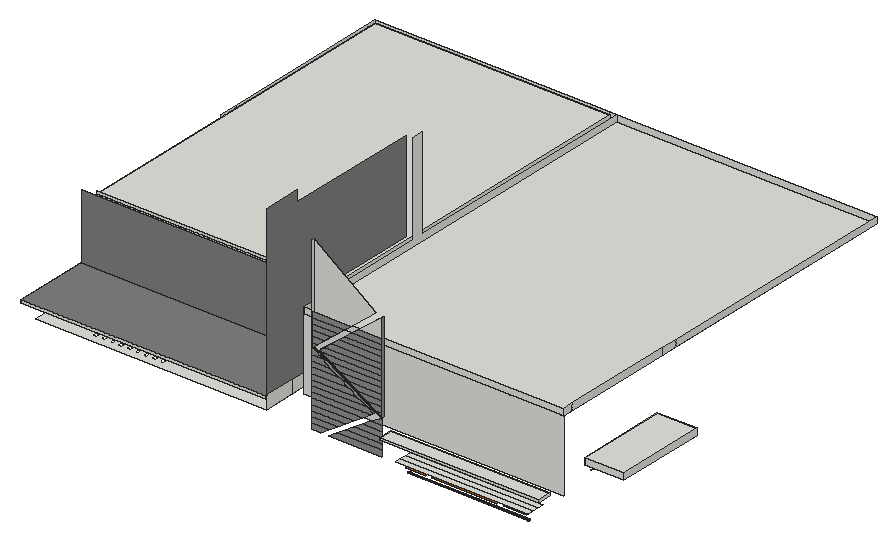
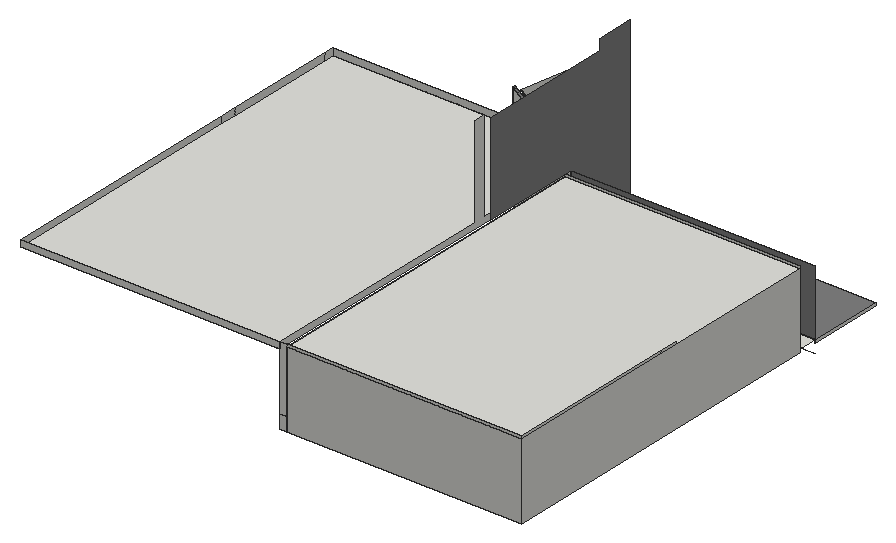
# SketchUp Ruby script. Lengths in inches.
U = 1.inch
M = Sketchup.active_model
def pt(a) = Geom::Point3d.new(a.map { |v| v * U })
def face(e, loops, mat)
  f = e.add_face(loops[0].map { |a| pt(a) })
  loops[1..].each { |l| e.add_face(l.map { |a| pt(a) }).erase! }
  f.material = f.back_material = mat if mat
  f
end
# faces: each face lists its corners as indices into pts; further lists are holes
def faces(e, pts, list, mat = nil) = list.each { |f| face(e, (f[0].is_a?(Array) ? f : [f]).map { |l| l.map { |i| pts[i] } }, mat) }
# xy, xz, yz: faces in a plane at the given z, y or x. An outline is a flat list of corners, or four numbers for a rectangle; further outlines are holes
def ring(l) = l.size == 4 ? [[l[0], l[1]], [l[2], l[1]], [l[2], l[3]], [l[0], l[3]]] : l.each_slice(2).to_a
def flat(e, list, mat, &to3) = list.each { |f| face(e, (f[0].is_a?(Array) ? f : [f]).map { |l| ring(l).map { |u, v| to3.(u, v) } }, mat) }
def xy(e, z, list, mat = nil) = flat(e, list, mat) { |x, y| [x, y, z] }
def xz(e, y, list, mat = nil) = flat(e, list, mat) { |x, z| [x, y, z] }
def yz(e, x, list, mat = nil) = flat(e, list, mat) { |y, z| [x, y, z] }
def lines(e, pts, list) = list.each { |a, b| e.add_line(pt(pts[a]), pt(pts[b])) }
# prism: a flat outline (further loops are holes) pulled along v
def prism(e, loops, v, mat = nil)
  f = face(e, loops, mat); d = Geom::Vector3d.new(v.map { |x| x * U })
  f.pushpull(f.normal.samedirection?(d) ? d.length : -d.length)
end
def box(e, o, s, mat = nil) = prism(e, [[o, [o[0] + s[0], o[1], o[2]], [o[0] + s[0], o[1] + s[1], o[2]], [o[0], o[1] + s[1], o[2]]]], [0, 0, s[2]], mat)
def at(x, y, z, deg = 0) = Geom::Transformation.translation(pt([x, y, z])) * Geom::Transformation.rotation(ORIGIN, Z_AXIS, deg.degrees)
def axes(o, x, y, z) = Geom::Transformation.new([*x, 0, *y, 0, *z, 0, *pt(o).to_a, 1])
def part(name) = M.definitions.add(name)
# library, detail: a bought-in or finely detailed component or shape, given as its bounding box
def library(name, o, s) = part(name).tap { |d| box(d.entities, o, s) }
def detail(e, o, s) = box(e.add_group.entities, o, s)
def put(e, d, t, mat = nil) = e.add_instance(d, t).tap { |i| i.material = mat if mat }
def group(e, t, mat = nil) = e.add_group.tap { |g| g.transformation = t; g.material = mat if mat }.entities
root = M.entities
M.materials.add("[0132_LightGray]").color = [169, 169, 169]
M.materials.add("[0133_Gray]").color = [128, 128, 128]
M.materials.add("[Color M04]").color = [142, 142, 142]
M.materials.add("[Wood Bamboo]").color = [195, 96, 5]
xy(root,318.58,[[351.24,38.65,369.24,44.67],[375.24,38.65,435.1,44.67],[441.1,38.65,462.7,44.67]],"[Wood Bamboo]")
xy(root,323.97,[[345.84,33.25,468.09,38.65],[345.84,38.65,468.09,44.67],[345.84,44.67,468.09,50.6875]])
xy(root,337.75,[[332.44,31.5625,478.87,33.25],[332.44,33.25,333.13,44.6875],[333.13,33.25,478.31,44.6875],[478.31,33.25,478.87,44.6875]])
xy(root,338,[[[28.03,15.6875,241.25,84.25],[55.53,37.52,56.5625,37.65,57.53,38.05,58.36,38.6875,58.99,39.52,59.39,40.48,59.53,41.52,59.39,42.55,58.99,43.52,58.36,44.34,57.53,44.98,56.5625,45.38,55.53,45.52,54.49,45.38,53.53,44.98,52.7,44.34,52.0625,43.52,51.66,42.55,51.53,41.52,51.66,40.48,52.0625,39.52,52.7,38.6875,53.53,38.05,54.49,37.65],[198.34,37.52,199.375,37.65,200.34,38.05,201.17,38.6875,201.8,39.52,202.2,40.48,202.34,41.52,202.2,42.55,201.8,43.52,201.17,44.34,200.34,44.98,199.375,45.38,198.34,45.52,197.31,45.38,196.34,44.98,195.51,44.34,194.875,43.52,194.48,42.55,194.34,41.52,194.48,40.48,194.875,39.52,195.51,38.6875,196.34,38.05,197.31,37.65],[74.77,23.01,78.7,26.95],[82.52,23.01,86.45,26.95],[90.27,23.01,94.2,26.95],[98.02,23.01,101.95,26.95],[105.77,23.01,109.7,26.95],[113.52,23.01,117.45,26.95],[121.27,23.01,125.2,26.95],[129.02,23.01,132.95,26.95],[136.77,23.01,140.7,26.95]],[55.53,37.52,54.49,37.65,53.53,38.05,52.7,38.6875,52.0625,39.52,51.66,40.48,51.53,41.52,51.66,42.55,52.0625,43.52,52.7,44.34,53.53,44.98,54.49,45.38,55.53,45.52,56.5625,45.38,57.53,44.98,58.36,44.34,58.99,43.52,59.39,42.55,59.53,41.52,59.39,40.48,58.99,39.52,58.36,38.6875,57.53,38.05,56.5625,37.65],[198.34,37.52,197.31,37.65,196.34,38.05,195.51,38.6875,194.875,39.52,194.48,40.48,194.34,41.52,194.48,42.55,194.875,43.52,195.51,44.34,196.34,44.98,197.31,45.38,198.34,45.52,199.375,45.38,200.34,44.98,201.17,44.34,201.8,43.52,202.2,42.55,202.34,41.52,202.2,40.48,201.8,39.52,201.17,38.6875,200.34,38.05,199.375,37.65]])
xy(root,339.8125,[[332.44,31.5625,478.87,44.6875]])
xy(root,347,[[14.875,14.6875,14.875,84.25,15.875,84.25,15.875,15.6875,241.25,15.6875,241.25,14.6875]])
xy(root,350,[[14.875,14.6875,241.25,84.25]],"[0133_Gray]")
xy(root,354,[[495.875,70.375,496.875,140.375]])
xy(root,361,[[495.875,63.375,496.875,147.375],[[496.875,63.375,531.875,147.375],[514.17,93.74,515.73,93.95,517.17,94.55,518.42,95.5,519.37,96.74,519.97,98.1875,520.17,99.74,519.97,101.3,519.37,102.74,518.42,103.98,517.17,104.9375,515.73,105.54,514.17,105.74,512.62,105.54,511.17,104.9375,509.93,103.98,508.98,102.74,508.375,101.3,508.17,99.74,508.375,98.1875,508.98,96.74,509.93,95.5,511.17,94.55,512.62,93.95]],[514.17,93.74,512.62,93.95,511.17,94.55,509.93,95.5,508.98,96.74,508.375,98.1875,508.17,99.74,508.375,101.3,508.98,102.74,509.93,103.98,511.17,104.9375,512.62,105.54,514.17,105.74,515.73,105.54,517.17,104.9375,518.42,103.98,519.37,102.74,519.97,101.3,520.17,99.74,519.97,98.1875,519.37,96.74,518.42,95.5,517.17,94.55,515.73,93.95]])
xy(root,367,[[495.875,63.375,531.875,147.375]])
xy(root,404,[[247.25,50.6875,486.875,411]])
xy(root,407.75,[[24.875,90.25,241.25,411]])
xz(root,14.6875,[[14.875,347,241.25,350]])
xz(root,31.5625,[[332.44,337.75,478.87,339.8125]])
xz(root,42.75,[[261.37,317.04,269.28,317.04,276.97,322.17,261.37,322.17],[276.6875,317.04,325.49,317.04,325.49,322.17,284.48,322.17],[261.37,322.17,276.97,322.17,284.66,327.29,261.37,327.29],[284.48,322.17,325.49,322.17,325.49,327.29,292.26,327.29],[261.37,327.29,284.66,327.29,292.35,332.42,261.37,332.42],
  [292.26,327.29,325.49,327.29,325.49,332.42,300.05,332.42],[261.37,332.42,292.35,332.42,300.04,337.54,261.37,337.54],[300.05,332.42,325.49,332.42,325.49,337.54,307.84,337.54],[261.37,337.54,300.04,337.54,307.73,342.67,261.37,342.67],[307.84,337.54,325.49,337.54,325.49,342.67,315.63,342.67],
  [261.37,342.67,307.73,342.67,315.42,347.79,261.37,347.79],[315.63,342.67,325.49,342.67,325.49,347.79,323.42,347.79],[261.37,347.79,315.42,347.79,317.38,349.1,311.37,352.92,261.37,352.92],[323.42,347.79,325.49,347.79,325.49,349.15],[325.49,349.15,325.49,352.92,319.41,352.92],
  [261.37,352.92,311.37,352.92,303.28,358.04,261.37,358.04],[319.41,352.92,325.49,352.92,325.49,358.04,311.14,358.04],[261.37,358.04,303.28,358.04,295.19,363.17,261.37,363.17],[311.14,358.04,325.49,358.04,325.49,363.17,302.875,363.17],[261.37,363.17,295.19,363.17,287.1,368.29,261.37,368.29],
  [302.875,363.17,325.49,363.17,325.49,368.29,294.61,368.29],[261.37,368.29,287.1,368.29,279.02,373.42,261.37,373.42],[294.61,368.29,325.49,368.29,325.49,373.42,286.34,373.42],[261.37,373.42,279.02,373.42,270.93,378.54,261.37,378.54],[286.34,373.42,325.49,373.42,325.49,378.54,278.07,378.54],
  [261.37,378.54,270.93,378.54,262.84,383.67,261.37,383.67],[278.07,378.54,325.49,378.54,325.49,383.67,269.8,383.67],[261.37,383.67,262.84,383.67,261.37,384.6],[269.8,383.67,325.49,383.67,325.49,388.79,273.37,388.79,268.3,384.6],[261.37,384.6,266.38,388.79,261.37,388.79],
  [261.37,388.79,266.38,388.79,272.51,393.92,261.37,393.92],[273.37,388.79,325.49,388.79,325.49,393.92,279.58,393.92],[261.37,393.92,272.51,393.92,278.64,399.04,261.37,399.04],[279.58,393.92,325.49,393.92,325.49,399.04,285.78,399.04],[261.37,399.04,278.64,399.04,284.76,404.17,261.37,404.17],
  [285.78,399.04,325.49,399.04,325.49,404.17,291.99,404.17],[261.37,404.17,284.76,404.17,290.89,409.29,261.37,409.29],[291.99,404.17,325.49,404.17,325.49,409.29,298.19,409.29],[261.37,409.29,290.89,409.29,297.02,414.42,261.37,414.42],[298.19,409.29,325.49,409.29,325.49,414.42,304.39,414.42]],"[Color M04]")
xz(root,44.6875,[[332.44,337.75,478.87,339.8125],[325.49,349.15,268.3,384.6,325.49,431.84],[261.37,384.6,261.37,473.32,318.21,432.15]])
xz(root,50.6875,[[247.25,338,486.875,404],[247.25,404,486.875,410]])
xz(root,63.375,[[495.875,361,531.875,367]])
xz(root,84.25,[[14.875,347,15.875,350]])
xz(root,84.25,[[15.875,350,241.25,410]],"[0133_Gray]")
xz(root,90.25,[[24.875,338,241.25,407.75],[24.875,407.75,241.25,410]])
xz(root,147.375,[[495.875,361,531.875,367]])
xz(root,411,[[24.875,338,241.25,407.75],[241.25,338,247.25,350],[241.25,350,247.25,410],[247.25,404,486.875,410],[24.875,407.75,241.25,410]])
yz(root,14.875,[[14.6875,347,84.25,350]])
yz(root,24.875,[[90.25,338,411,407.75],[233.22,407.75,250.625,410],[250.625,407.75,411,410]])
yz(root,241.25,[[15.6875,338,44.6875,350],[44.6875,338,84.25,350],[90.25,338,411,407.75],[14.6875,347,15.6875,350]])
yz(root,241.25,[[15.6875,350,15.6875,503.875,50.6875,503.875,50.6875,494,176.25,494,176.25,410,84.25,410,84.25,350]],"[0133_Gray]")
yz(root,247.25,[[50.6875,404,411,404,411,410,187,410,187,494,176.25,494,176.25,410,50.6875,410]])
yz(root,261.37,[[42.75,384.6,44.6875,473.32]])
yz(root,325.49,[[42.75,349.15,44.6875,431.84]],"[Color M04]")
yz(root,332.44,[[31.5625,337.75,44.6875,339.8125]])
yz(root,478.87,[[31.5625,337.75,44.6875,339.8125]])
yz(root,486.875,[[50.6875,404,60.17,410],[60.17,404,163.89,410],[163.89,404,180.07,410],[180.07,404,411,410]])
yz(root,495.875,[[63.375,361,147.375,367]])
yz(root,531.875,[[63.375,361,147.375,367]])
p = [[351.24,41.41,313.07],[351.24,41.53,313.02],[462.7,41.53,313.02],[462.7,41.41,313.07],[351.24,41.66,313.01],[462.7,41.66,313.01],
  [351.24,41.31,313.15],[462.7,41.31,313.15],[351.24,41.23,313.26],[462.7,41.23,313.26],[351.24,41.18,313.375],[462.7,41.18,313.375],
  [351.24,41.16,313.51],[462.7,41.16,313.51],[351.24,41.18,313.63],[462.7,41.18,313.63],[351.24,41.23,313.76],[462.7,41.23,313.76],
  [351.24,41.31,313.86],[462.7,41.31,313.86],[351.24,41.41,313.9375],[462.7,41.41,313.9375],[351.24,41.53,313.99],[462.7,41.53,313.99],
  [351.24,41.66,314.01],[462.7,41.66,314.01],[317.38,44.6875,349.1],[261.37,44.6875,384.6],[261.37,42.75,384.6],[262.84,42.75,383.67],
  [270.93,42.75,378.54],[279.02,42.75,373.42],[287.1,42.75,368.29],[295.19,42.75,363.17],[303.28,42.75,358.04],[311.37,42.75,352.92],
  [317.38,42.75,349.1],[268.3,44.6875,384.6],[325.49,44.6875,349.15],[325.49,42.75,349.15],[319.41,42.75,352.92],[311.14,42.75,358.04],
  [302.875,42.75,363.17],[294.61,42.75,368.29],[286.34,42.75,373.42],[278.07,42.75,378.54],[269.8,42.75,383.67],[268.3,42.75,384.6],
  [318.21,44.6875,432.15],[318.21,42.75,432.15],[315.4,42.75,429.79],[309.27,42.75,424.67],[303.14,42.75,419.54],[297.02,42.75,414.42],
  [290.89,42.75,409.29],[284.76,42.75,404.17],[278.64,42.75,399.04],[272.51,42.75,393.92],[266.38,42.75,388.79],[325.49,44.6875,431.84],
  [273.37,42.75,388.79],[279.58,42.75,393.92],[285.78,42.75,399.04],[291.99,42.75,404.17],[298.19,42.75,409.29],[304.39,42.75,414.42],
  [310.6,42.75,419.54],[316.8,42.75,424.67],[323.01,42.75,429.79],[325.49,42.75,431.84],[15.875,84.25,338],[28.03,84.25,338]]
faces(root,p,[[0,1,2,3],[1,4,5,2],[6,0,3,7],[8,6,7,9],[10,8,9,11],[12,10,11,13],[14,12,13,15],[16,14,15,17],
  [18,16,17,19],[20,18,19,21],[22,20,21,23],[24,22,23,25]],"[0132_LightGray]")
faces(root,p,[[26,27,28,29,30,31,32,33,34,35,36],[37,38,39,40,41,42,43,44,45,46,47],[27,48,49,50,51,52,53,54,55,56,57,58,28],[59,37,47,60,61,62,63,64,65,66,67,68,69]],"[Color M04]")
lines(root,p,[[70,71]])
